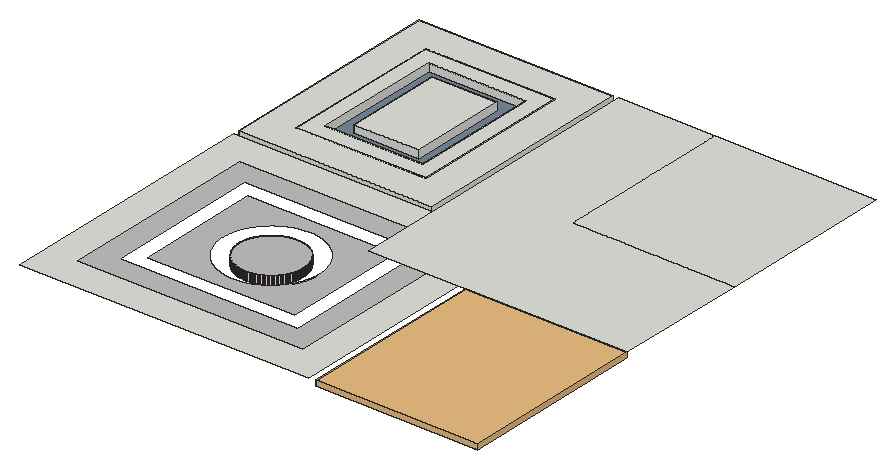
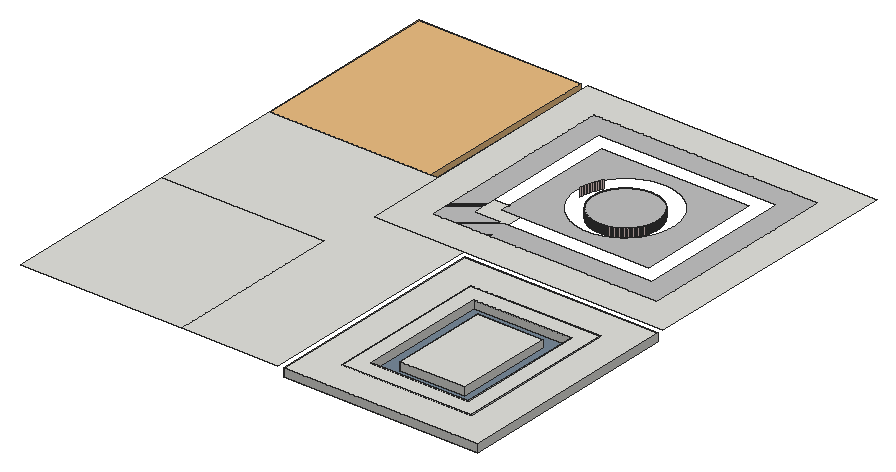
# SketchUp Ruby script. Lengths in inches.
U = 1.inch
M = Sketchup.active_model
def pt(a) = Geom::Point3d.new(a.map { |v| v * U })
def face(e, loops, mat)
  f = e.add_face(loops[0].map { |a| pt(a) })
  loops[1..].each { |l| e.add_face(l.map { |a| pt(a) }).erase! }
  f.material = f.back_material = mat if mat
  f
end
# faces: each face lists its corners as indices into pts; further lists are holes
def faces(e, pts, list, mat = nil) = list.each { |f| face(e, (f[0].is_a?(Array) ? f : [f]).map { |l| l.map { |i| pts[i] } }, mat) }
# xy, xz, yz: faces in a plane at the given z, y or x. An outline is a flat list of corners, or four numbers for a rectangle; further outlines are holes
def ring(l) = l.size == 4 ? [[l[0], l[1]], [l[2], l[1]], [l[2], l[3]], [l[0], l[3]]] : l.each_slice(2).to_a
def flat(e, list, mat, &to3) = list.each { |f| face(e, (f[0].is_a?(Array) ? f : [f]).map { |l| ring(l).map { |u, v| to3.(u, v) } }, mat) }
def xy(e, z, list, mat = nil) = flat(e, list, mat) { |x, y| [x, y, z] }
def xz(e, y, list, mat = nil) = flat(e, list, mat) { |x, z| [x, y, z] }
def yz(e, x, list, mat = nil) = flat(e, list, mat) { |y, z| [x, y, z] }
def lines(e, pts, list) = list.each { |a, b| e.add_line(pt(pts[a]), pt(pts[b])) }
# prism: a flat outline (further loops are holes) pulled along v
def prism(e, loops, v, mat = nil)
  f = face(e, loops, mat); d = Geom::Vector3d.new(v.map { |x| x * U })
  f.pushpull(f.normal.samedirection?(d) ? d.length : -d.length)
end
def box(e, o, s, mat = nil) = prism(e, [[o, [o[0] + s[0], o[1], o[2]], [o[0] + s[0], o[1] + s[1], o[2]], [o[0], o[1] + s[1], o[2]]]], [0, 0, s[2]], mat)
def at(x, y, z, deg = 0) = Geom::Transformation.translation(pt([x, y, z])) * Geom::Transformation.rotation(ORIGIN, Z_AXIS, deg.degrees)
def axes(o, x, y, z) = Geom::Transformation.new([*x, 0, *y, 0, *z, 0, *pt(o).to_a, 1])
def part(name) = M.definitions.add(name)
# library, detail: a bought-in or finely detailed component or shape, given as its bounding box
def library(name, o, s) = part(name).tap { |d| box(d.entities, o, s) }
def detail(e, o, s) = box(e.add_group.entities, o, s)
def put(e, d, t, mat = nil) = e.add_instance(d, t).tap { |i| i.material = mat if mat }
def group(e, t, mat = nil) = e.add_group.tap { |g| g.transformation = t; g.material = mat if mat }.entities
root = M.entities
M.materials.add("[0007_MistyRose]").color = [255, 228, 225]
M.materials.add("[0110_LightSlateGray]").color = [119, 136, 153]
M.materials.add("[0131_Silver]").color = [192, 192, 192]
c1 = library("Group\#42",[0,0,-4],[120.75,139.5,4])
xy(root,120,[[[9,107.25,224.75,306.75],[33,131.25,200.75,282.75]],[158.21,246.75,351,246.75,351,347.25,230.25,347.25,230.25,480,158.21,480],[230.25,347.25,351,480]])
xy(root,120,[[[33,131.25,200.75,282.75],[50.24,148.49,183.51,265.51]],[[62.05,160.3,171.7,253.7],[116.7,171,117.83,171.01,118.96,171.0625,120.09,171.14,121.21,171.26,122.33,171.42,123.45,171.61,124.56,171.83,125.66,172.09,126.75,172.38,127.83,172.71,128.91,173.07,129.97,173.46,131.01,173.89,132.05,174.35,133.0625,174.85,134.07,175.37,135.05,175.92,136.02,176.51,136.97,177.13,137.89,177.77,138.8,178.45,139.6875,179.15,140.55,179.88,141.39,180.64,142.21,181.42,143,182.23,143.76,183.0625,144.5,183.92,145.21,184.8,145.9,185.7,146.55,186.62,147.18,187.5625,147.77,188.52,148.34,189.5,148.87,190.5,149.375,191.51,149.84,192.54,150.28,193.59,150.6875,194.64,151.06,195.71,151.4,196.79,151.7,197.88,151.97,198.98,152.2,200.08,152.4,201.2,152.57,202.32,152.7,203.4375,152.79,204.57,152.85,205.7,152.875,206.83,152.86,207.96,152.8125,209.09,152.73,210.21,152.61,211.34,152.46,212.46,152.27,213.57,152.05,214.68,151.79,215.78,151.49,216.875,151.17,217.96,150.81,219.03,150.41,220.09,149.98,221.14,149.52,222.17,149.03,223.1875,148.51,224.19,147.95,225.18,147.36,226.14,146.75,227.09,146.1,228.02,145.43,228.93,144.72,229.8125,143.99,230.68,143.24,231.52,142.45,232.33,141.65,233.125,140.8125,233.89,139.96,234.63,139.08,235.34,138.18,236.02,137.25,236.68,136.3125,237.3,135.35,237.9,134.37,238.46,133.375,239,132.36,239.5,131.33,239.97,130.29,240.41,129.23,240.8125,128.17,241.18,127.09,241.52,126,241.83,124.9,242.09,123.79,242.33,122.68,242.53,121.56,242.69,120.4375,242.82,119.31,242.92,118.18,242.98,117.05,243,115.92,242.99,114.79,242.9375,113.66,242.86,112.54,242.74,111.42,242.58,110.3,242.39,109.19,242.17,108.09,241.91,107,241.62,105.92,241.29,104.84,240.93,103.78,240.54,102.74,240.11,101.7,239.65,100.6875,239.15,99.68,238.63,98.7,238.08,97.73,237.49,96.78,236.87,95.86,236.23,94.95,235.55,94.0625,234.85,93.2,234.12,92.36,233.36,91.54,232.58,90.75,231.77,89.99,230.9375,89.25,230.08,88.54,229.2,87.85,228.3,87.2,227.38,86.57,226.4375,85.98,225.48,85.41,224.5,84.88,223.5,84.375,222.49,83.91,221.46,83.47,220.41,83.0625,219.36,82.69,218.29,82.35,217.21,82.05,216.12,81.78,215.02,81.55,213.92,81.35,212.8,81.18,211.68,81.05,210.5625,80.96,209.43,80.9,208.3,80.875,207.17,80.89,206.04,80.9375,204.91,81.02,203.79,81.14,202.66,81.29,201.54,81.48,200.43,81.7,199.32,81.96,198.22,82.26,197.125,82.58,196.04,82.94,194.97,83.34,193.91,83.77,192.86,84.23,191.83,84.72,190.8125,85.24,189.81,85.8,188.82,86.39,187.86,87,186.91,87.65,185.98,88.32,185.07,89.03,184.1875,89.76,183.32,90.51,182.48,91.3,181.67,92.1,180.875,92.9375,180.11,93.79,179.37,94.67,178.66,95.57,177.98,96.5,177.32,97.4375,176.7,98.4,176.1,99.38,175.54,100.375,175,101.39,174.5,102.42,174.03,103.46,173.59,104.52,173.1875,105.58,172.82,106.66,172.48,107.75,172.17,108.85,171.91,109.96,171.67,111.07,171.47,112.19,171.31,113.3125,171.18,114.44,171.08,115.57,171.02]],[116.59,183,115.83,183.02,115.08,183.07,114.33,183.14,113.58,183.23,112.84,183.34,112.1,183.48,111.36,183.64,110.63,183.83,109.9,184.03,109.1875,184.27,108.48,184.52,107.77,184.79,107.08,185.09,106.4,185.41,105.72,185.75,105.0625,186.11,104.41,186.49,103.77,186.89,103.15,187.3125,102.54,187.75,101.9375,188.21,101.36,188.69,100.79,189.1875,100.24,189.7,99.7,190.23,99.18,190.78,98.68,191.35,98.2,191.92,97.74,192.52,97.29,193.125,96.86,193.75,96.46,194.38,96.07,195.03,95.71,195.69,95.36,196.36,95.04,197.04,94.74,197.73,94.46,198.43,94.2,199.14,93.96,199.86,93.75,200.58,93.56,201.31,93.39,202.05,93.25,202.79,93.13,203.53,93.03,204.28,92.96,205.03,92.91,205.78,92.88,206.53,92.875,207.29,92.9,208.04,92.94,208.79,93.01,209.54,93.1,210.29,93.22,211.04,93.36,211.78,93.52,212.52,93.7,213.25,93.91,213.97,94.14,214.6875,94.39,215.4,94.67,216.1,94.96,216.79,95.28,217.48,95.62,218.15,95.98,218.8125,96.36,219.46,96.77,220.1,97.1875,220.73,97.63,221.34,98.09,221.9375,98.57,222.52,99.0625,223.09,99.58,223.64,100.11,224.17,100.66,224.69,101.22,225.19,101.8,225.67,102.39,226.14,103,226.58,103.625,227.01,104.26,227.42,104.91,227.8,105.57,228.17,106.24,228.51,106.92,228.84,107.61,229.14,108.31,229.42,109.02,229.68,109.73,229.91,110.46,230.125,111.19,230.32,111.92,230.48,112.66,230.63,113.4,230.75,114.15,230.85,114.9,230.92,115.65,230.97,116.41,231,117.16,231,117.92,230.98,118.67,230.93,119.42,230.86,120.17,230.77,120.91,230.66,121.65,230.52,122.39,230.36,123.12,230.17,123.85,229.97,124.5625,229.73,125.27,229.48,125.98,229.21,126.67,228.91,127.35,228.59,128.03,228.25,128.6875,227.89,129.34,227.51,129.98,227.11,130.6,226.6875,131.21,226.25,131.8125,225.79,132.39,225.31,132.96,224.8125,133.51,224.3,134.05,223.77,134.57,223.22,135.07,222.65,135.55,222.08,136.01,221.48,136.46,220.875,136.89,220.25,137.29,219.62,137.68,218.97,138.04,218.31,138.39,217.64,138.71,216.96,139.01,216.27,139.29,215.57,139.55,214.86,139.79,214.14,140,213.42,140.19,212.69,140.36,211.95,140.5,211.21,140.62,210.47,140.72,209.72,140.79,208.97,140.84,208.22,140.87,207.47,140.875,206.71,140.85,205.96,140.81,205.21,140.74,204.46,140.65,203.71,140.53,202.96,140.39,202.22,140.23,201.48,140.05,200.75,139.84,200.03,139.61,199.3125,139.36,198.6,139.08,197.9,138.79,197.21,138.47,196.52,138.13,195.85,137.77,195.1875,137.39,194.54,136.98,193.9,136.5625,193.27,136.12,192.66,135.66,192.0625,135.18,191.48,134.6875,190.91,134.17,190.36,133.64,189.83,133.09,189.31,132.53,188.81,131.95,188.33,131.36,187.86,130.75,187.42,130.125,186.99,129.49,186.58,128.84,186.2,128.18,185.83,127.51,185.49,126.83,185.16,126.14,184.86,125.44,184.58,124.73,184.32,124.02,184.09,123.29,183.875,122.56,183.68,121.83,183.52,121.09,183.37,120.35,183.25,119.6,183.15,118.85,183.08,118.1,183.03,117.34,183]],"[0131_Silver]")
xz(root,183,[[116.59,114,117.34,120]],"[0007_MistyRose]")
xz(root,231,[[116.41,114,117.16,120]],"[0007_MistyRose]")
p = [[115.08,183.07,120],[115.83,183.02,120],[115.83,183.02,114],[115.08,183.07,114],[116.59,183,120],[116.59,183,114],
  [117.34,183,120],[118.1,183.03,120],[118.1,183.03,114],[117.34,183,114],[118.85,183.08,120],[118.85,183.08,114],
  [113.58,183.23,120],[114.33,183.14,120],[114.33,183.14,114],[113.58,183.23,114],[119.6,183.15,120],[119.6,183.15,114],
  [112.84,183.34,120],[112.84,183.34,114],[120.35,183.25,120],[120.35,183.25,114],[112.1,183.48,120],[112.1,183.48,114],
  [121.09,183.37,120],[121.09,183.37,114],[121.83,183.52,120],[121.83,183.52,114],[111.36,183.64,120],[111.36,183.64,114],
  [122.56,183.68,120],[122.56,183.68,114],[110.63,183.83,120],[110.63,183.83,114],[123.29,183.875,120],[123.29,183.875,114],
  [109.9,184.03,120],[109.9,184.03,114],[124.02,184.09,120],[124.02,184.09,114],[109.1875,184.27,120],[109.1875,184.27,114],
  [124.73,184.32,120],[124.73,184.32,114],[108.48,184.52,120],[108.48,184.52,114],[125.44,184.58,120],[125.44,184.58,114],
  [107.77,184.79,120],[107.77,184.79,114],[126.14,184.86,120],[126.14,184.86,114],[107.08,185.09,120],[107.08,185.09,114],
  [126.83,185.16,120],[126.83,185.16,114],[106.4,185.41,120],[106.4,185.41,114],[127.51,185.49,120],[127.51,185.49,114],
  [105.72,185.75,120],[105.72,185.75,114],[128.18,185.83,120],[128.18,185.83,114],[105.0625,186.11,120],[105.0625,186.11,114],
  [128.84,186.2,120],[128.84,186.2,114],[104.41,186.49,120],[104.41,186.49,114],[129.49,186.58,120],[129.49,186.58,114],
  [103.77,186.89,120],[103.77,186.89,114],[130.125,186.99,120],[130.125,186.99,114],[103.15,187.3125,120],[103.15,187.3125,114],
  [130.75,187.42,120],[130.75,187.42,114],[102.54,187.75,120],[102.54,187.75,114],[131.36,187.86,120],[131.36,187.86,114],
  [101.9375,188.21,120],[101.9375,188.21,114],[131.95,188.33,120],[131.95,188.33,114],[101.36,188.69,120],[101.36,188.69,114],
  [132.53,188.81,120],[132.53,188.81,114],[148.34,189.5,120],[147.77,188.52,120],[147.77,188.52,114],[148.34,189.5,114],
  [100.79,189.1875,120],[100.79,189.1875,114],[133.09,189.31,120],[133.09,189.31,114],[100.24,189.7,120],[100.24,189.7,114],
  [133.64,189.83,120],[133.64,189.83,114],[148.87,190.5,120],[148.87,190.5,114],[99.7,190.23,120],[99.7,190.23,114],
  [134.17,190.36,120],[134.17,190.36,114],[99.18,190.78,120],[99.18,190.78,114],[134.6875,190.91,120],[134.6875,190.91,114],
  [149.375,191.51,120],[149.375,191.51,114],[98.68,191.35,120],[98.68,191.35,114],[135.18,191.48,120],[135.18,191.48,114],
  [98.2,191.92,120],[98.2,191.92,114],[135.66,192.0625,120],[135.66,192.0625,114],[149.84,192.54,120],[149.84,192.54,114],
  [97.74,192.52,120],[97.74,192.52,114],[136.12,192.66,120],[136.12,192.66,114],[97.29,193.125,120],[97.29,193.125,114],
  [150.28,193.59,120],[150.28,193.59,114],[136.5625,193.27,120],[136.5625,193.27,114],[96.86,193.75,120],[96.86,193.75,114],
  [136.98,193.9,120],[136.98,193.9,114],[150.6875,194.64,120],[150.6875,194.64,114],[96.46,194.38,120],[96.46,194.38,114],
  [137.39,194.54,120],[137.39,194.54,114],[96.07,195.03,120],[96.07,195.03,114],[137.77,195.1875,120],[137.77,195.1875,114],
  [151.06,195.71,120],[151.06,195.71,114],[95.71,195.69,120],[95.71,195.69,114],[138.13,195.85,120],[138.13,195.85,114],
  [95.36,196.36,120],[95.36,196.36,114],[151.4,196.79,120],[151.4,196.79,114],[138.47,196.52,120],[138.47,196.52,114],
  [95.04,197.04,120],[95.04,197.04,114],[138.79,197.21,120],[138.79,197.21,114],[151.7,197.88,120],[151.7,197.88,114],
  [94.74,197.73,120],[94.74,197.73,114],[139.08,197.9,120],[139.08,197.9,114],[94.46,198.43,120],[94.46,198.43,114],
  [139.36,198.6,120],[139.36,198.6,114],[151.97,198.98,120],[151.97,198.98,114],[94.2,199.14,120],[94.2,199.14,114],
  [139.61,199.3125,120],[139.61,199.3125,114],[152.2,200.08,120],[152.2,200.08,114],[93.96,199.86,120],[93.96,199.86,114],
  [139.84,200.03,120],[139.84,200.03,114],[93.75,200.58,120],[93.75,200.58,114],[140.05,200.75,120],[140.05,200.75,114],
  [152.4,201.2,120],[152.4,201.2,114],[93.56,201.31,120],[93.56,201.31,114],[140.23,201.48,120],[140.23,201.48,114],
  [152.57,202.32,120],[152.57,202.32,114],[93.39,202.05,120],[93.39,202.05,114],[140.39,202.22,120],[140.39,202.22,114],
  [93.25,202.79,120],[93.25,202.79,114],[140.53,202.96,120],[140.53,202.96,114],[152.7,203.4375,120],[152.7,203.4375,114],
  [93.13,203.53,120],[93.13,203.53,114],[140.65,203.71,120],[140.65,203.71,114],[152.79,204.57,120],[152.79,204.57,114],
  [93.03,204.28,120],[93.03,204.28,114],[140.74,204.46,120],[140.74,204.46,114],[92.96,205.03,120],[92.96,205.03,114],
  [140.81,205.21,120],[140.81,205.21,114],[92.91,205.78,120],[92.91,205.78,114],[140.85,205.96,120],[140.85,205.96,114],
  [92.88,206.53,120],[92.88,206.53,114],[140.875,206.71,120],[140.875,206.71,114],[92.875,207.29,120],[92.875,207.29,114],
  [140.87,207.47,120],[140.87,207.47,114],[92.9,208.04,120],[92.9,208.04,114],[140.84,208.22,120],[140.84,208.22,114],
  [92.94,208.79,120],[92.94,208.79,114],[140.79,208.97,120],[140.79,208.97,114],[93.01,209.54,120],[93.01,209.54,114],
  [140.72,209.72,120],[140.72,209.72,114],[93.1,210.29,120],[93.1,210.29,114],[140.62,210.47,120],[140.62,210.47,114],
  [93.22,211.04,120],[93.22,211.04,114],[140.5,211.21,120],[140.5,211.21,114],[93.36,211.78,120],[93.36,211.78,114],
  [140.36,211.95,120],[140.36,211.95,114],[93.52,212.52,120],[93.52,212.52,114],[140.19,212.69,120],[140.19,212.69,114],
  [93.7,213.25,120],[93.7,213.25,114],[140,213.42,120],[140,213.42,114],[93.91,213.97,120],[93.91,213.97,114],
  [139.79,214.14,120],[139.79,214.14,114],[94.14,214.6875,120],[94.14,214.6875,114],[139.55,214.86,120],[139.55,214.86,114],
  [94.39,215.4,120],[94.39,215.4,114],[139.29,215.57,120],[139.29,215.57,114],[94.67,216.1,120],[94.67,216.1,114],
  [139.01,216.27,120],[139.01,216.27,114],[94.96,216.79,120],[94.96,216.79,114],[138.71,216.96,120],[138.71,216.96,114],
  [95.28,217.48,120],[95.28,217.48,114],[138.39,217.64,120],[138.39,217.64,114],[95.62,218.15,120],[95.62,218.15,114],
  [138.04,218.31,120],[138.04,218.31,114],[95.98,218.8125,120],[95.98,218.8125,114],[137.68,218.97,120],[137.68,218.97,114],
  [96.36,219.46,120],[96.36,219.46,114],[137.29,219.62,120],[137.29,219.62,114],[96.77,220.1,120],[96.77,220.1,114],
  [136.89,220.25,120],[136.89,220.25,114],[97.1875,220.73,120],[97.1875,220.73,114],[136.46,220.875,120],[136.46,220.875,114],
  [97.63,221.34,120],[97.63,221.34,114],[136.01,221.48,120],[136.01,221.48,114],[98.09,221.9375,120],[98.09,221.9375,114],
  [135.55,222.08,120],[135.55,222.08,114],[98.57,222.52,120],[98.57,222.52,114],[135.07,222.65,120],[135.07,222.65,114],
  [99.0625,223.09,120],[99.0625,223.09,114],[134.57,223.22,120],[134.57,223.22,114],[99.58,223.64,120],[99.58,223.64,114],
  [134.05,223.77,120],[134.05,223.77,114],[100.11,224.17,120],[100.11,224.17,114],[133.51,224.3,120],[133.51,224.3,114],
  [100.66,224.69,120],[100.66,224.69,114],[132.96,224.8125,120],[132.96,224.8125,114],[101.22,225.19,120],[101.22,225.19,114],
  [132.39,225.31,120],[132.39,225.31,114],[101.8,225.67,120],[101.8,225.67,114],[131.8125,225.79,120],[131.8125,225.79,114],
  [102.39,226.14,120],[102.39,226.14,114],[131.21,226.25,120],[131.21,226.25,114],[103,226.58,120],[103,226.58,114],
  [130.6,226.6875,120],[130.6,226.6875,114],[103.625,227.01,120],[103.625,227.01,114],[129.98,227.11,120],[129.98,227.11,114],
  [104.26,227.42,120],[104.26,227.42,114],[129.34,227.51,120],[129.34,227.51,114],[104.91,227.8,120],[104.91,227.8,114],
  [128.6875,227.89,120],[128.6875,227.89,114],[105.57,228.17,120],[105.57,228.17,114],[128.03,228.25,120],[128.03,228.25,114],
  [106.24,228.51,120],[106.24,228.51,114],[127.35,228.59,120],[127.35,228.59,114],[106.92,228.84,120],[106.92,228.84,114],
  [126.67,228.91,120],[126.67,228.91,114],[107.61,229.14,120],[107.61,229.14,114],[125.98,229.21,120],[125.98,229.21,114],
  [108.31,229.42,120],[108.31,229.42,114],[125.27,229.48,120],[125.27,229.48,114],[109.02,229.68,120],[109.02,229.68,114],
  [124.5625,229.73,120],[124.5625,229.73,114],[109.73,229.91,120],[109.73,229.91,114],[123.85,229.97,120],[123.85,229.97,114],
  [110.46,230.125,120],[110.46,230.125,114],[123.12,230.17,120],[123.12,230.17,114],[111.19,230.32,120],[111.19,230.32,114],
  [122.39,230.36,120],[122.39,230.36,114],[111.92,230.48,120],[111.92,230.48,114],[121.65,230.52,120],[121.65,230.52,114],
  [112.66,230.63,120],[112.66,230.63,114],[120.91,230.66,120],[120.91,230.66,114],[113.4,230.75,120],[113.4,230.75,114],
  [114.15,230.85,120],[114.15,230.85,114],[120.17,230.77,120],[120.17,230.77,114],[114.9,230.92,120],[114.9,230.92,114],
  [119.42,230.86,120],[119.42,230.86,114],[115.65,230.97,120],[115.65,230.97,114],[118.67,230.93,120],[117.92,230.98,120],
  [117.92,230.98,114],[118.67,230.93,114],[116.41,231,120],[116.41,231,114],[117.16,231,120],[117.16,231,114]]
faces(root,p,[[0,1,2,3],[1,4,5,2],[6,7,8,9],[7,10,11,8],[12,13,14,15],[13,0,3,14],[10,16,17,11],[18,12,15,19],
  [16,20,21,17],[22,18,19,23],[20,24,25,21],[24,26,27,25],[28,22,23,29],[26,30,31,27],[32,28,29,33],[30,34,35,31],
  [36,32,33,37],[34,38,39,35],[40,36,37,41],[38,42,43,39],[44,40,41,45],[42,46,47,43],[48,44,45,49],[46,50,51,47],
  [52,48,49,53],[50,54,55,51],[56,52,53,57],[54,58,59,55],[60,56,57,61],[58,62,63,59],[64,60,61,65],[62,66,67,63],
  [68,64,65,69],[66,70,71,67],[72,68,69,73],[70,74,75,71],[76,72,73,77],[74,78,79,75],[80,76,77,81],[78,82,83,79],
  [84,80,81,85],[82,86,87,83],[88,84,85,89],[86,90,91,87],[92,93,94,95],[96,88,89,97],[90,98,99,91],[100,96,97,101],
  [98,102,103,99],[104,92,95,105],[106,100,101,107],[102,108,109,103],[110,106,107,111],[108,112,113,109],[114,104,105,115],[116,110,111,117],
  [112,118,119,113],[120,116,117,121],[118,122,123,119],[124,114,115,125],[126,120,121,127],[122,128,129,123],[130,126,127,131],[132,124,125,133],
  [128,134,135,129],[136,130,131,137],[134,138,139,135],[140,132,133,141],[142,136,137,143],[138,144,145,139],[146,142,143,147],[144,148,149,145],
  [150,140,141,151],[152,146,147,153],[148,154,155,149],[156,152,153,157],[158,150,151,159],[154,160,161,155],[162,156,157,163],[160,164,165,161],
  [166,158,159,167],[168,162,163,169],[164,170,171,165],[172,168,169,173],[170,174,175,171],[176,166,167,177],[178,172,173,179],[174,180,181,175],
  [182,176,177,183],[184,178,179,185],[180,186,187,181],[188,184,185,189],[186,190,191,187],[192,182,183,193],[194,188,189,195],[190,196,197,191],
  [198,192,193,199],[200,194,195,201],[196,202,203,197],[204,200,201,205],[202,206,207,203],[208,198,199,209],[210,204,205,211],[206,212,213,207],
  [214,208,209,215],[216,210,211,217],[212,218,219,213],[220,216,217,221],[218,222,223,219],[224,220,221,225],[222,226,227,223],[228,224,225,229],
  [226,230,231,227],[232,228,229,233],[230,234,235,231],[236,232,233,237],[234,238,239,235],[240,236,237,241],[238,242,243,239],[244,240,241,245],
  [242,246,247,243],[248,244,245,249],[246,250,251,247],[252,248,249,253],[250,254,255,251],[256,252,253,257],[254,258,259,255],[260,256,257,261],
  [258,262,263,259],[264,260,261,265],[262,266,267,263],[268,264,265,269],[266,270,271,267],[272,268,269,273],[270,274,275,271],[276,272,273,277],
  [274,278,279,275],[280,276,277,281],[278,282,283,279],[284,280,281,285],[282,286,287,283],[288,284,285,289],[286,290,291,287],[292,288,289,293],
  [290,294,295,291],[296,292,293,297],[294,298,299,295],[300,296,297,301],[298,302,303,299],[304,300,301,305],[302,306,307,303],[308,304,305,309],
  [306,310,311,307],[312,308,309,313],[310,314,315,311],[316,312,313,317],[314,318,319,315],[320,316,317,321],[318,322,323,319],[324,320,321,325],
  [322,326,327,323],[328,324,325,329],[326,330,331,327],[332,328,329,333],[330,334,335,331],[336,332,333,337],[334,338,339,335],[340,336,337,341],
  [338,342,343,339],[344,340,341,345],[342,346,347,343],[348,344,345,349],[346,350,351,347],[352,348,349,353],[350,354,355,351],[356,352,353,357],
  [354,358,359,355],[360,356,357,361],[358,362,363,359],[364,360,361,365],[362,366,367,363],[368,364,365,369],[366,370,371,367],[372,368,369,373],
  [370,374,375,371],[376,372,373,377],[374,378,379,375],[380,376,377,381],[378,382,383,379],[384,380,381,385],[382,386,387,383],[388,384,385,389],
  [386,390,391,387],[392,388,389,393],[390,394,395,391],[396,392,393,397],[394,398,399,395],[400,396,397,401],[398,402,403,399],[404,400,401,405],
  [402,406,407,403],[408,404,405,409],[406,410,411,407],[412,408,409,413],[414,412,413,415],[410,416,417,411],[418,414,415,419],[416,420,421,417],
  [422,418,419,423],[424,425,426,427],[420,424,427,421],[428,422,423,429],[425,430,431,426]],"[0007_MistyRose]")
g1 = group(root,at(9,311.25,120))
xy(g1,-6,[[[0,0,144.75,168.75],[24,24,120.75,144.75]],[[36,36,108.75,132.75],[48,48,96.75,120.75]]],"[0110_LightSlateGray]")
xy(g1,0,[[[0,0,144.75,168.75],[24,24,120.75,144.75]],[[24,24,120.75,144.75],[36,36,108.75,132.75]],[48,48,96.75,120.75]])
xz(g1,0,[[0,-6,144.75,0]])
xz(g1,24,[[24,-6,120.75,0]])
xz(g1,36,[[36,-6,108.75,0]])
xz(g1,48,[[48,-6,96.75,0]])
xz(g1,120.75,[[48,-6,96.75,0]])
xz(g1,132.75,[[36,-6,108.75,0]])
xz(g1,144.75,[[24,-6,120.75,0]])
xz(g1,168.75,[[0,-6,144.75,0]])
yz(g1,0,[[0,-6,168.75,0]])
yz(g1,24,[[24,-6,144.75,0]])
yz(g1,36,[[36,-6,132.75,0]])
yz(g1,48,[[48,-6,120.75,0]])
yz(g1,96.75,[[48,-6,120.75,0]])
yz(g1,108.75,[[36,-6,132.75,0]])
yz(g1,120.75,[[24,-6,144.75,0]])
yz(g1,144.75,[[0,-6,168.75,0]])
put(root,c1,at(230.25,107.25,120))
